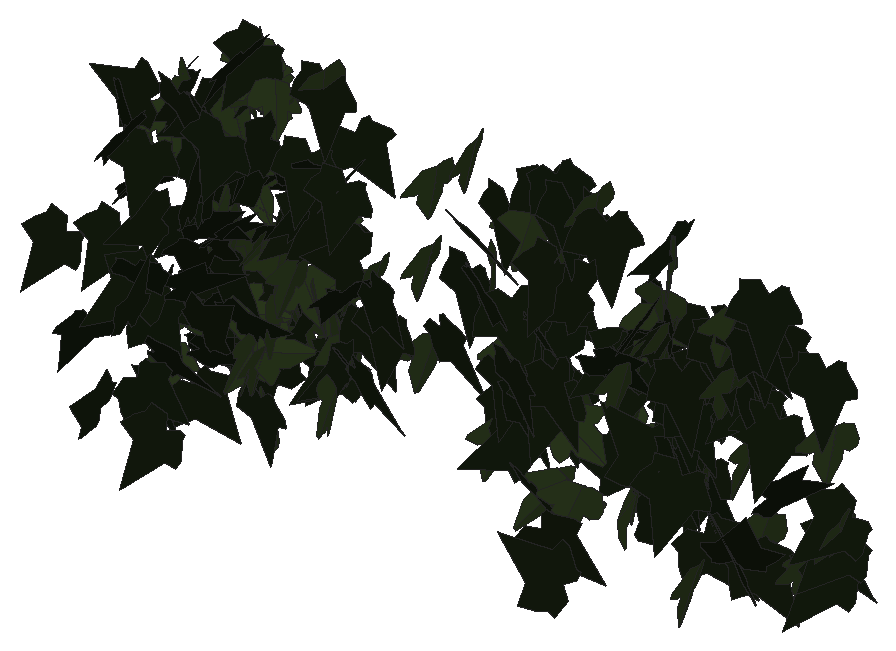
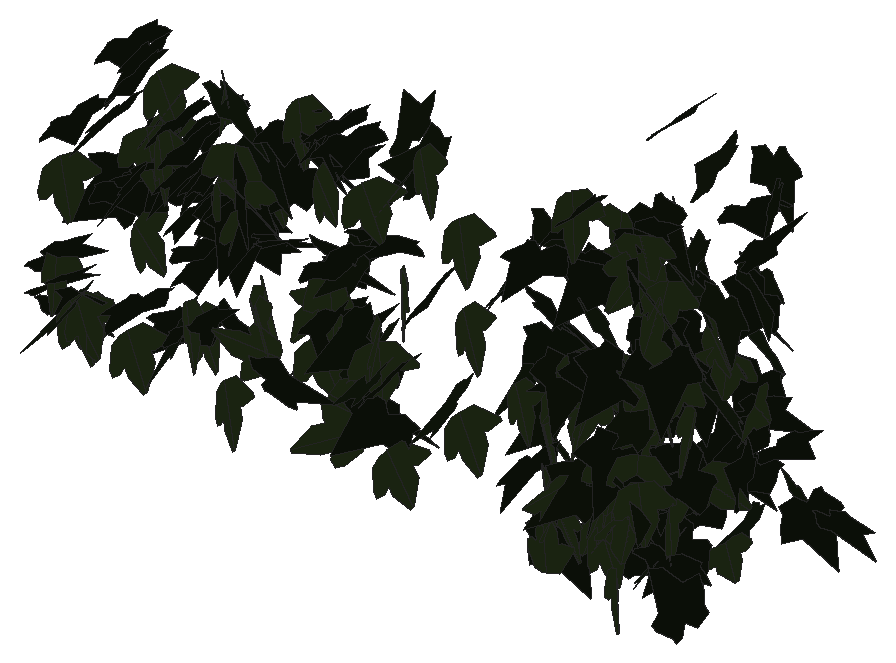
# SketchUp Ruby script. Lengths in inches.
U = 1.inch
M = Sketchup.active_model
def pt(a) = Geom::Point3d.new(a.map { |v| v * U })
def face(e, loops, mat)
  f = e.add_face(loops[0].map { |a| pt(a) })
  loops[1..].each { |l| e.add_face(l.map { |a| pt(a) }).erase! }
  f.material = f.back_material = mat if mat
  f
end
# faces: each face lists its corners as indices into pts; further lists are holes
def faces(e, pts, list, mat = nil) = list.each { |f| face(e, (f[0].is_a?(Array) ? f : [f]).map { |l| l.map { |i| pts[i] } }, mat) }
# xy, xz, yz: faces in a plane at the given z, y or x. An outline is a flat list of corners, or four numbers for a rectangle; further outlines are holes
def ring(l) = l.size == 4 ? [[l[0], l[1]], [l[2], l[1]], [l[2], l[3]], [l[0], l[3]]] : l.each_slice(2).to_a
def flat(e, list, mat, &to3) = list.each { |f| face(e, (f[0].is_a?(Array) ? f : [f]).map { |l| ring(l).map { |u, v| to3.(u, v) } }, mat) }
def xy(e, z, list, mat = nil) = flat(e, list, mat) { |x, y| [x, y, z] }
def xz(e, y, list, mat = nil) = flat(e, list, mat) { |x, z| [x, y, z] }
def yz(e, x, list, mat = nil) = flat(e, list, mat) { |y, z| [x, y, z] }
def lines(e, pts, list) = list.each { |a, b| e.add_line(pt(pts[a]), pt(pts[b])) }
# prism: a flat outline (further loops are holes) pulled along v
def prism(e, loops, v, mat = nil)
  f = face(e, loops, mat); d = Geom::Vector3d.new(v.map { |x| x * U })
  f.pushpull(f.normal.samedirection?(d) ? d.length : -d.length)
end
def box(e, o, s, mat = nil) = prism(e, [[o, [o[0] + s[0], o[1], o[2]], [o[0] + s[0], o[1] + s[1], o[2]], [o[0], o[1] + s[1], o[2]]]], [0, 0, s[2]], mat)
def at(x, y, z, deg = 0) = Geom::Transformation.translation(pt([x, y, z])) * Geom::Transformation.rotation(ORIGIN, Z_AXIS, deg.degrees)
def axes(o, x, y, z) = Geom::Transformation.new([*x, 0, *y, 0, *z, 0, *pt(o).to_a, 1])
def part(name) = M.definitions.add(name)
# library, detail: a bought-in or finely detailed component or shape, given as its bounding box
def library(name, o, s) = part(name).tap { |d| box(d.entities, o, s) }
def detail(e, o, s) = box(e.add_group.entities, o, s)
def put(e, d, t, mat = nil) = e.add_instance(d, t).tap { |i| i.material = mat if mat }
def group(e, t, mat = nil) = e.add_group.tap { |g| g.transformation = t; g.material = mat if mat }.entities
root = M.entities
M.materials.add("efeu1").color = [18, 25, 13]
M.materials.add("efeu2").color = [43, 57, 29]
c1 = part("ivyleaf_9")
p = [[1.54,2.16,1.25],[1.36,2.04,1.19],[-0.21,0.99,0.68],[-0.71,1.11,0.82],[-0.85,0.86,0.67],[-0.8,0.17,0.21],
  [-0.9,-0.01,0.1],[-0.67,-0.16,-0.02],[-0.08,-0.08,-0.05],[-0.03,-0.6,-0.4],[0.65,-0.88,-0.66],[0.83,-0.6,-0.49],
  [1.29,-0.42,-0.43],[1.8125,-0.07,-0.26],[1.21,0.44,0.15]]
faces(c1.entities,p,[[0,1,2,3,4,5,6,7,8,9,10,11,12,13,14]],"efeu1")
c2 = part("ivyleaf_10")
p = [[0,0.5,-0.03],[-0.0625,2.02,-0.43],[-0.19,2.01,-0.46],[-0.54,1.05,-0.29],[-0.52,0.625,-0.18],[-0.83,0.76,-0.28],
  [-1.16,0.64,-0.33],[-1.15,0.33,-0.24],[-0.77,-0.39,0.02],[-0.3,-0.51,0.16],[0.04,-0.48,0.23],[-0.02,2.01,-0.4375],
  [-0.06,2.01,-0.43],[0.04,-0.49,0.23],[0.67,-0.49,0.14],[1.38,0.36,-0.2],[1.375,0.51,-0.24],[0.81,0.65,-0.19],
  [0.62,0.59,-0.15],[0.6,1.09,-0.28],[0.5,1.23,-0.31]]
faces(c2.entities,p,[[0,1,2,3,4,5,6,7,8,9,10],[11,12,0,13,14,15,16,17,18,19,20]],"efeu2")
put(root,c1,axes([2.38,221.57,243.66],[-0.44883,-0.12115,-0.04461],[0.04538,0.00913,-0.45018],[0.13117,-0.41769,0.0031]))
put(root,c2,axes([3.58,222.25,245.79],[-0.02282,0.31345,-0.31292],[-0.01067,-0.3015,-0.32594],[-0.46912,-0.00839,0.02263]))
put(root,c1,axes([3.82,220.47,242.92],[-0.00565,0.32008,-0.30631],[0.01893,-0.29415,-0.33279],[-0.46938,-0.01571,-0.00974]))
put(root,c1,axes([3.92,221.19,244.42],[-0.23643,-0.35754,0.12069],[-0.05224,-0.10638,-0.43577],[0.4026,-0.22377,0.01433]))
put(root,c2,axes([4.58,222.32,246.94],[-0.13824,0.10281,0.41894],[-0.42529,0.10517,-0.15805],[-0.14397,-0.40938,0.06461]))
put(root,c2,axes([4.21,222.22,246.49],[0.43273,0.13992,0.09924],[0.09551,0.03618,-0.44135],[-0.156,0.41029,0.00508]))
put(root,c1,axes([4.64,221.82,247.36],[-0.08663,0.41338,0.1135],[-0.02945,0.10586,-0.43788],[-0.4608,-0.08448,0.00665]))
put(root,c1,axes([4.85,221.9,247.14],[-0.29901,0.33234,0.04787],[-0.02666,0.03934,-0.44981],[-0.36138,-0.27789,-0.00643]))
put(root,c1,axes([4.93,220.75,247.68],[-0.07576,-0.41549,-0.11238],[0.01633,-0.11181,0.43692],[-0.46336,0.06399,0.03377]))
put(root,c1,axes([4.46,223.21,241.59],[-0.00786,-0.11862,0.48566],[0.37542,-0.32217,-0.07261],[0.33015,0.36351,0.09413]))
put(root,c1,axes([5.16,219.1,242.17],[-0.24445,0.31807,0.19958],[-0.11,0.16297,-0.40586],[-0.38582,-0.24798,-0.01074]))
put(root,c2,axes([4.87,221.46,242.12],[0.18139,0.37992,-0.1343],[-0.05106,-0.12028,-0.43197],[-0.43035,0.17441,-0.00535]))
put(root,c1,axes([5.08,220.65,243.03],[-0.00146,-0.05257,0.44908],[0.14124,0.41179,0.05256],[-0.44806,0.12998,0.0151]))
put(root,c2,axes([4.97,222.91,243.27],[0.16507,-0.45863,0.11138],[0.16192,-0.05581,-0.46975],[0.44332,0.19116,0.1301]))
put(root,c1,axes([5.42,221.15,244.96],[-0.17381,0.37113,0.28645],[-0.22198,0.20393,-0.39892],[-0.41293,-0.26585,0.09387]))
put(root,c1,axes([5.3125,220.32,244.26],[-0.39403,-0.23092,0.2035],[-0.18567,-0.08533,-0.45634],[0.24549,-0.43519,-0.01851]))
put(root,c1,axes([4.93,223,242.6],[-0.24815,-0.29365,-0.31968],[0.27813,0.17515,-0.37679],[0.33327,-0.36482,0.07641]))
put(root,c2,axes([5.35,221.4,243.29],[0.1724,0.23306,-0.34403],[-0.33805,-0.15425,-0.27011],[-0.27697,0.33334,0.11554]))
put(root,c2,axes([5.12,222.6875,246.01],[-0.43543,-0.20452,-0.13628],[0.13098,0.04149,-0.48075],[0.20795,-0.45437,0.01745]))
put(root,c1,axes([5.28,222.67,246.39],[0.2811,0.35236,-0.2164],[-0.1876,-0.12452,-0.44643],[-0.3685,0.33218,0.0622]))
put(root,c2,axes([5.31,221.98,244.75],[-0.36612,0.32316,0.10736],[-0.08834,0.06211,-0.4882],[-0.32887,-0.37645,0.01162]))
put(root,c1,axes([5.3125,219.49,248.31],[0.26102,-0.08163,-0.36644],[-0.34839,0.14299,-0.26457],[0.17664,0.40264,0.01967]))
put(root,c1,axes([5.25,220.01,246.49],[0.18079,0.35094,0.20286],[0.09269,0.17517,-0.40437],[-0.4236,0.18811,-0.00191]))
put(root,c1,axes([5.5,219.74,246.71],[-0.09877,0.40443,0.13678],[-0.04326,0.12574,-0.43108],[-0.45726,-0.09925,0.01124]))
put(root,c2,axes([5.41,222.99,246.74],[-0.41969,0.19074,-0.04447],[-0.03985,0.02186,0.4502],[0.20732,0.39034,-0.00348]))
put(root,c1,axes([5.08,220.61,242.03],[0.28274,-0.34,0.07419],[0.04798,-0.05583,-0.44627],[0.37211,0.26554,0.00117]))
put(root,c1,axes([5.7,221.52,247.35],[-0.39604,0.29621,0.07354],[-0.08253,0.01206,-0.49299],[-0.29384,-0.40263,0.03935]))
put(root,c2,axes([5.48,223.19,243.73],[-0.28716,-0.34197,0.04141],[-0.02624,-0.03155,-0.4505],[0.37089,-0.267,0.00019]))
put(root,c1,axes([5.38,219.92,244.75],[0.37325,0.22216,-0.14864],[-0.13716,-0.06663,-0.4271],[-0.25016,0.36801,0.0124]))
put(root,c1,axes([5.28,222.01,242.37],[0.41846,0.19665,0.0215],[0.01597,0.01653,-0.45181],[-0.21295,0.38766,0.00836]))
put(root,c1,axes([5.31,220.42,243.72],[0.11413,-0.39475,-0.28486],[-0.08978,0.2705,-0.41082],[0.47845,0.14492,-0.00913]))
put(root,c1,axes([5.24,221.92,243.76],[0.43877,0.19884,0.13397],[0.12528,0.04809,-0.48166],[-0.20443,0.45624,-0.00762]))
put(root,c1,axes([5.23,222.85,242.47],[0.21399,-0.45177,-0.01042],[0.01905,0.02054,-0.49921],[0.45149,0.21326,0.026]))
put(root,c1,axes([5.68,222.74,243.79],[0.02488,0.42017,0.11464],[0.00053,0.11036,-0.4376],[-0.46914,0.02241,0.00559]))
put(root,c2,axes([5.65,223.05,244.18],[-0.34054,-0.2963,-0.04661],[0.02608,0.03972,-0.44981],[0.32259,-0.316,-0.01283]))
put(root,c2,axes([5.78,223.55,242.04],[-0.32013,0.27253,0.17116],[-0.20236,0.03247,-0.40688],[-0.27799,-0.33748,0.09907]))
put(root,c1,axes([5.95,222.47,247.48],[-0.2793,0.2882,0.20614],[-0.14473,0.14606,-0.4027],[-0.34894,-0.29126,0.00203]))
put(root,c2,axes([5.66,222.22,247.33],[-0.23266,-0.43515,-0.08068],[0.1725,-0.00522,-0.46927],[0.40757,-0.2462,0.15255]))
put(root,c1,axes([6.04,219.6875,246.06],[-0.42437,0.15774,0.10372],[-0.09989,0.0373,-0.44035],[-0.17506,-0.40367,-0.00016]))
put(root,c1,axes([5.98,222.08,243.18],[-0.29202,-0.11745,0.33267],[-0.26024,-0.22283,-0.29692],[0.26021,-0.35465,0.07639]))
put(root,c1,axes([5.7,219.59,242.71],[0.05768,-0.17441,-0.41071],[-0.04482,0.394,-0.18681],[0.46409,0.05973,0.033]))
put(root,c1,axes([6.04,220.82,245.02],[0.18318,0.34092,-0.21872],[-0.1369,-0.17097,-0.39455],[-0.41039,0.20921,0.03399]))
put(root,c1,axes([6.11,218.57,248.33],[-0.12026,0.41668,-0.05882],[0.0159,-0.05461,-0.44856],[-0.45387,-0.11233,-0.00013]))
put(root,c2,axes([6,221.93,245.03],[0.30728,-0.32039,-0.07801],[-0.04546,0.06291,-0.4455],[0.35246,0.28743,0.01055]))
put(root,c2,axes([5.74,222.63,245.54],[0.37507,0.10251,0.2507],[0.25048,0.06573,-0.37658],[-0.1315,0.41761,-0.00226]))
put(root,c1,axes([6.31,221.93,242.65],[-0.37067,0.2467,0.10694],[-0.108,0.03667,-0.43863],[-0.26768,-0.3564,0.02889]))
put(root,c1,axes([6.1,221.75,243.6],[0.19313,0.37256,-0.14126],[-0.08671,-0.1119,-0.42913],[-0.4194,0.1947,0.02367]))
put(root,c1,axes([6.01,223.09,244.4],[0.25845,0.36319,-0.00739],[-0.00273,-0.00685,-0.45234],[-0.39231,0.23931,-0.00173]))
put(root,c2,axes([6.08,221.41,245.81],[0.35729,-0.26353,-0.10571],[-0.08777,0.06111,-0.43987],[0.29215,0.34065,-0.00287]))
put(root,c1,axes([5.77,222.62,245.06],[0.49392,-0.07764,0.0039],[0.02128,0.11091,-0.48708],[0.07476,0.48132,0.11287]))
put(root,c2,axes([6.01,222.41,248.33],[0.4375,0.15631,-0.02734],[-0.02266,-0.01864,-0.45146],[-0.16968,0.40552,-0.01022]))
put(root,c1,axes([6.17,218.6875,244.54],[-0.32584,0.29805,-0.10065],[-0.08951,0.05366,0.44059],[0.32639,0.31227,0.02035]))
put(root,c2,axes([6.02,222.76,243.86],[-0.29111,0.33396,-0.07384],[0.04583,-0.05699,-0.44632],[-0.36588,-0.27285,0.00284]))
put(root,c2,axes([6.01,222.84,242.83],[0.16973,0.4053,0.01674],[0.00762,0.01453,-0.45209],[-0.438,0.15731,-0.00138]))
put(root,c1,axes([5.79,221.28,247.45],[0.26936,-0.3165,0.1704],[0.11017,-0.12822,-0.41908],[0.36881,0.26946,0.00073]))
put(root,c1,axes([6.29,221.76,248.57],[-0.20377,0.39759,-0.2245],[0.04549,-0.22694,-0.4432],[-0.45432,-0.20105,0.05632]))
put(root,c2,axes([6.08,222.44,244.23],[-0.10898,0.03132,-0.43885],[-0.02759,-0.43347,-0.02711],[-0.45615,0.01873,0.10648]))
put(root,c1,axes([6.48,221.93,243.47],[-0.29718,0.04316,0.3475],[-0.35892,0.03607,-0.28948],[-0.05975,-0.43135,0.01056]))
put(root,c1,axes([5.88,223.34,243.11],[0.18161,-0.40114,0.006],[0.00559,-0.00409,-0.45235],[0.43324,0.1682,0.00332]))
put(root,c2,axes([6.03,221.69,245.33],[-0.07319,-0.17005,0.41039],[0.18267,-0.37779,-0.1391],[0.4266,0.1326,0.12998]))
put(root,c1,axes([6.26,221.77,246.08],[-0.06048,0.15389,-0.41912],[0.04269,-0.40284,-0.16569],[-0.46393,-0.05713,0.03939]))
put(root,c1,axes([6.11,219.34,247.69],[-0.23779,-0.37229,-0.04821],[0.02855,0.03822,-0.44981],[0.40417,-0.22173,0.00341]))
put(root,c1,axes([6.27,222.46,247.33],[0.15373,-0.09716,0.41538],[-0.127,0.39538,0.14361],[-0.42538,-0.15316,0.10724]))
put(root,c2,axes([6.2,223.05,244.05],[-0.35389,-0.28311,-0.04292],[0.03555,0.02502,-0.45035],[0.30693,-0.32932,0.00267]))
put(root,c1,axes([5.84,219.93,243.15],[0.39874,-0.10404,0.21337],[0.21232,-0.05873,-0.39891],[0.12899,0.41827,-0.00294]))
put(root,c1,axes([6.27,222.29,248.47],[-0.33067,-0.30723,0.03434],[-0.02376,-0.02469,-0.45109],[0.33287,-0.30696,0.00192]))
put(root,c2,axes([6.15,222.3,247.73],[-0.34812,-0.23113,-0.27458],[0.2434,0.12908,-0.41725],[0.26376,-0.42417,0.02264]))
put(root,c1,axes([6.18,220.75,246.96],[-0.31354,-0.12197,-0.31212],[0.32512,0.04729,-0.32284],[0.12924,-0.41486,0.05496]))
put(root,c1,axes([6.52,222.39,241.75],[0.15282,-0.00661,0.42774],[-0.43864,0.06664,0.14644],[-0.07035,-0.42981,0.01613]))
put(root,c1,axes([6.24,222.3,246.71],[-0.14105,0.07933,-0.42357],[0.3248,-0.27607,-0.15622],[-0.30874,-0.32668,0.02916]))
put(root,c1,axes([6.14,220.63,242.28],[-0.01518,-0.22267,-0.38836],[0.06952,0.36844,-0.231],[0.46438,-0.06244,0.02189]))
put(root,c2,axes([6.21,222.19,248.01],[0.27029,0.32136,0.15882],[0.11244,0.11239,-0.42342],[-0.36744,0.27078,-0.01274]))
put(root,c1,axes([6.25,220.61,245.63],[0.32435,0.28092,0.1475],[0.10275,0.10583,-0.42751],[-0.32396,0.31482,0.01209]))
put(root,c1,axes([6.07,220.92,242.88],[0.38112,0.06429,0.25593],[0.25443,0.07604,-0.372],[-0.10355,0.42345,0.02794]))
put(root,c1,axes([6.28,221.27,244.57],[0.27768,-0.25959,-0.24552],[-0.15187,0.19191,-0.37874],[0.34719,0.29156,0.0307]))
put(root,c2,axes([6.47,222.92,242.41],[-0.06303,-0.48642,0.09706],[0.01069,-0.09915,-0.48995],[0.4959,-0.05969,0.0229]))
put(root,c1,axes([6.57,219.17,242.15],[-0.44393,-0.13934,-0.03035],[0.03094,0.00639,-0.45137],[0.15061,-0.41203,0.00326]))
put(root,c1,axes([6.52,222.86,243.82],[0.21707,-0.04547,-0.39842],[-0.37121,0.17506,-0.20915],[0.18921,0.39562,0.04676]))
put(root,c1,axes([6.35,222.65,245.77],[0.32123,0.30332,0.09732],[0.06492,0.07209,-0.44174],[-0.33661,0.30336,0.00767]))
put(root,c1,axes([6.39,220.98,245.28],[0.24152,0.27566,0.26151],[0.08751,0.25028,-0.36029],[-0.39335,0.22494,0.08042]))
put(root,c1,axes([6.59,219.85,246.31],[0.09615,0.06942,0.4369],[-0.05982,0.42742,-0.06125],[-0.45595,-0.04144,0.10017]))
put(root,c2,axes([6.54,222.48,244.24],[-0.22582,-0.37876,0.04704],[0.01017,-0.05668,-0.44844],[0.41184,-0.20628,0.03686]))
put(root,c1,axes([6.26,219.99,244.62],[0.266,0.10392,0.35689],[0.2955,0.2146,-0.27182],[-0.25027,0.36383,0.05838]))
put(root,c2,axes([6.4,222.92,242.79],[0.00165,0.00839,0.45231],[0.29431,-0.33902,0.00581],[0.36618,0.27244,-0.00671]))
put(root,c2,axes([6.6,222.98,242.92],[-0.43604,0.15085,-0.06117],[0.06291,-0.01213,-0.44815],[-0.16316,-0.40783,-0.0093]))
put(root,c1,axes([6.37,219.89,248.57],[0.17828,-0.41207,0.22003],[0.12183,-0.18634,-0.4477],[0.45097,0.21324,0.03396]))
put(root,c2,axes([6.4,221.55,243.53],[0.04472,-0.12992,-0.4296],[0.4659,0.04843,0.02913],[0.04064,-0.41231,0.13879]))
put(root,c1,axes([6.58,220.3,243.72],[-0.11605,0.00969,0.43826],[0.31469,-0.31254,0.08475],[0.32896,0.3024,0.07354]))
put(root,c2,axes([6.93,221.16,242.87],[0.18226,-0.33228,-0.23333],[-0.0802,0.2133,-0.38664],[0.42551,0.18253,0.02706]))
put(root,c1,axes([6.77,220.08,246.54],[-0.10135,0.26328,0.34665],[0.07605,-0.32699,0.28923],[0.45239,0.11396,0.02904]))
put(root,c1,axes([7.21,222.34,242.95],[-0.32925,0.30802,0.03898],[-0.03653,0.01925,-0.45059],[-0.33312,-0.30656,0.01087]))
put(root,c2,axes([6.98,221.17,243.05],[0.07198,0.26015,-0.35589],[-0.11568,-0.32532,-0.2789],[-0.44961,0.12535,0.01479]))
put(root,c1,axes([6.81,223.11,243.4375],[0.46214,0.0608,0.05116],[0.03965,0.08545,-0.44194],[-0.07459,0.42217,0.08208]))
put(root,c2,axes([7.15,221.52,241.25],[-0.19281,0.39223,-0.06158],[-0.0357,0.04999,0.44809],[0.42692,0.18132,0.00966]))
put(root,c2,axes([7.2,223.25,242.8125],[0.36347,-0.1958,-0.20173],[-0.16716,0.11903,-0.40426],[0.24629,0.36975,0.02332]))
put(root,c2,axes([7.15,221.2,243.03],[0.05432,-0.43206,0.00425],[0.00254,-0.00384,-0.45238],[0.46664,0.05032,0.00197]))
put(root,c1,axes([6.75,221.09,243.6],[0.13887,-0.16067,0.39858],[0.38466,-0.16407,-0.19581],[0.23122,0.36945,0.08638]))
put(root,c2,axes([7.04,221.69,248.11],[0.46397,0.00222,0.07104],[0.07267,0.06223,-0.44224],[-0.0129,0.43052,0.06356]))
put(root,c1,axes([7.41,221.08,247.53],[-0.44852,0.12231,-0.04406],[0.04253,-0.01624,-0.45023],[-0.13317,-0.41714,0.00461]))
put(root,c1,axes([7.43,222.37,245.43],[-0.45645,-0.08004,0.06738],[-0.07078,-0.00202,-0.44723],[0.08579,-0.42757,-0.0105]))
put(root,c2,axes([7.2,223.42,243.3],[0.13325,0.01563,-0.43352],[0.10594,0.42142,0.04663],[0.43787,-0.10671,0.12065]))
put(root,c1,axes([6.97,222.49,245.39],[0.15915,-0.03211,-0.42434],[0.14053,0.41483,0.01492],[0.41909,-0.12691,0.15614]))
put(root,c1,axes([7.05,221.34,242.01],[0.09256,-0.41008,0.12179],[0.05061,-0.10967,-0.43507],[0.4578,0.09504,0.02347]))
put(root,c2,axes([7.3,221.27,243.68],[0.11266,-0.17364,-0.40035],[0.00771,0.39719,-0.18432],[0.45603,0.03619,0.10202]))
put(root,c1,axes([7.51,222.96,242.2],[0.14356,0.2054,-0.37406],[-0.22457,-0.2936,-0.25429],[-0.38687,0.24665,0.0088]))
put(root,c2,axes([7.4375,222.5625,245.42],[-0.15753,-0.38954,0.13241],[-0.00522,-0.13349,-0.43054],[0.44257,-0.14023,0.04205]))
put(root,c1,axes([7.5,222.7,245.32],[0.096,0.41126,0.11481],[-0.00054,0.11288,-0.4369],[-0.45989,0.08572,0.02448]))
put(root,c2,axes([7.36,223.45,241.91],[-0.44783,0.03341,0.13222],[0.13689,-0.00996,0.43265],[0.03766,0.4336,-0.00025]))
put(root,c2,axes([7.24,221.3,243.09],[0.00702,-0.13365,-0.43046],[0.30107,0.31904,-0.10259],[0.36058,-0.26378,0.09404]))
put(root,c1,axes([7.76,222.99,242.28],[-0.43965,-0.11009,0.11098],[-0.10517,-0.04819,-0.43806],[0.1279,-0.41807,0.02127]))
put(root,c1,axes([7.8,221.65,246.05],[-0.34907,0.2911,-0.00456],[0.00359,-0.00286,-0.45238],[-0.3144,-0.32323,-0.00011]))
put(root,c2,axes([7.6,222.94,242.38],[-0.17744,0.3943,0.08553],[-0.02459,0.07959,-0.44413],[-0.43431,-0.1656,-0.0098]))
put(root,c2,axes([7.46,222.66,245.07],[0.25254,0.27149,0.25653],[0.1198,0.22649,-0.36861],[-0.37761,0.25342,0.05462]))
put(root,c2,axes([7.53,221.97,244.3],[0.23183,0.34724,0.15625],[0.03813,0.1536,-0.42166],[-0.40683,0.21227,0.04952]))
put(root,c2,axes([7.67,221.49,244.79],[-0.03288,-0.40682,0.15702],[0.02916,-0.15284,-0.42262],[0.46774,-0.01907,0.03739]))
put(root,c2,axes([7.6,222.82,243.22],[-0.10927,0.42292,-0.01172],[0.0032,-0.01088,-0.45225],[-0.4569,-0.10122,-0.00037]))
put(root,c2,axes([7.74,222.23,248.41],[-0.11326,-0.48158,-0.07247],[0.00618,0.07298,-0.49461],[0.48696,-0.11293,-0.01058]))
put(root,c2,axes([7.73,222.04,244.07],[-0.24509,0.35957,0.09551],[-0.07269,0.06599,-0.44165],[-0.39416,-0.23575,0.02206]))
put(root,c2,axes([7.74,222.2,245.04],[-0.44517,-0.12121,-0.07077],[0.06566,0.03431,-0.44654],[0.13501,-0.41636,-0.01619]))
put(root,c1,axes([7.65,221.55,246.78],[0.39545,0.22792,0.05892],[0.04438,0.04114,-0.44834],[-0.24973,0.36822,0.01362]))
put(root,c1,axes([7.96,221.97,245.72],[-0.45427,0.01655,-0.11408],[0.11496,-0.06084,-0.43406],[-0.03371,-0.43041,0.05697]))
put(root,c1,axes([7.71,222.37,248.24],[0.00576,-0.49847,0.03866],[0.00416,-0.03862,-0.49849],[0.49995,0.00606,0.0037]))
put(root,c1,axes([7.89,221.67,247.11],[-0.32256,-0.28007,-0.15279],[0.13867,0.07729,-0.4247],[0.31215,-0.32374,0.03078]))
put(root,c2,axes([7.94,222.77,244.05],[0.27789,-0.41497,-0.02415],[-0.00533,0.02549,-0.49932],[0.41563,0.27777,0.00975]))
put(root,c2,axes([7.875,222.49,242.91],[0.00413,-0.4268,0.08734],[0.14318,-0.07885,-0.423],[0.44743,0.02917,0.13455]))
put(root,c2,axes([8.08,222.58,242.91],[0.31848,-0.31,-0.08165],[-0.00103,0.10594,-0.43878],[0.34537,0.28618,0.07399]))
put(root,c1,axes([8.01,219.07,248.65],[-0.12399,-0.44497,0.19138],[0.05564,-0.20933,-0.45065],[0.48118,-0.09045,0.10143]))
put(root,c1,axes([8.14,222.93,243.41],[0.12414,-0.42358,-0.23488],[-0.04823,0.23046,-0.44109],[0.48194,0.13217,0.01636]))
put(root,c1,axes([8.67,221.625,243.08],[-0.39706,0.23151,0.0223],[-0.01956,0.01148,-0.45185],[-0.25034,-0.3681,-0.00007]))
put(root,c2,axes([8.49,222.82,244.54],[0.02585,-0.43422,-0.01054],[-0.01565,0.00934,-0.45204],[0.46883,0.02426,-0.01451]))
put(root,c1,axes([8.33,222.45,247.36],[-0.04597,-0.26031,-0.35974],[0.07533,0.33891,-0.27417],[0.46144,-0.08126,0.00892]))
put(root,c1,axes([9.15,221.41,245.56],[-0.33767,0.17792,0.25435],[-0.23557,0.11103,-0.374],[-0.22628,-0.3811,0.00979]))
put(root,c1,axes([8.98,221.25,244.93],[-0.02059,0.40693,-0.15863],[-0.06469,-0.15368,-0.41862],[-0.46487,0.00337,0.06528]))
put(root,c1,axes([9.02,221.22,247.16],[-0.17336,0.40402,0.01578],[-0.02317,0.00779,-0.45178],[-0.43603,-0.16105,0.01773]))
put(root,c1,axes([8.83,221.43,243.43],[0.4371,-0.15922,-0.00881],[-0.00841,0.00335,-0.45231],[0.172,0.4048,0.00028]))
put(root,c1,axes([9,221.28,247.06],[-0.14791,-0.40968,0.05338],[0.02748,-0.06235,-0.44695],[0.44506,-0.1323,0.04534]))
put(root,c2,axes([9.26,220.51,243.2],[0.34912,-0.33136,-0.13535],[-0.07727,0.11483,-0.48046],[0.34949,0.35639,0.02897]))
put(root,c2,axes([9.77,222.79,243.47],[-0.12928,-0.46601,0.12696],[-0.01658,-0.12707,-0.4833],[0.48271,-0.12917,0.0174]))
put(root,c2,axes([9.86,222.57,245.44],[0.04833,-0.49676,0.02984],[0.00137,-0.02985,-0.49911],[0.49766,0.04833,-0.00152]))
put(root,c1,axes([9.79,220.68,243.82],[0.4158,-0.23238,-0.15203],[-0.11449,0.10595,-0.47505],[0.253,0.42985,0.0349]))
put(root,c2,axes([10.07,222.49,247.15],[-0.09101,-0.49159,-0.00778],[-0.00197,0.00827,-0.49993],[0.49164,-0.09096,-0.00344]))
put(root,c1,axes([10.02,222.76,243.85],[0.34419,-0.3522,-0.08656],[-0.02583,0.09523,-0.49017],[0.36176,0.34189,0.04736]))
put(root,c1,axes([10.27,220.5,245.72],[0.33005,-0.3115,-0.20984],[-0.13793,0.1593,-0.45343],[0.34935,0.3572,0.01922]))
put(root,c1,axes([10.49,220.64,245.13],[-0.00698,-0.47016,0.17],[0.04622,-0.1699,-0.46797],[0.49781,0.00919,0.04584]))
put(root,c2,axes([11.08,222.29,248.125],[0.09954,-0.48817,-0.04219],[-0.00688,0.04166,-0.49821],[0.48994,0.09976,0.00158]))
put(root,c1,axes([10.93,222.42,245.5],[0.07453,-0.47612,0.13326],[0.00431,-0.13413,-0.48165],[0.4944,0.07294,-0.01589]))
put(root,c2,axes([11.32,222.88,242.22],[-0.14836,-0.43772,0.19075],[-0.00677,-0.1978,-0.45916],[0.47743,-0.13883,0.05276]))
put(root,c2,axes([11.29,222.6,245.74],[0.29351,-0.38472,-0.12586],[0.0105,0.16265,-0.47269],[0.40465,0.27483,0.10356]))
put(root,c2,axes([11.81,222.67,244.12],[-0.37902,-0.32159,0.05407],[0.03712,-0.12492,-0.48272],[0.32398,-0.36191,0.11857]))
put(root,c1,axes([11.52,222.83,243.08],[-0.04936,-0.16243,-0.4703],[0.25648,0.39667,-0.16392],[0.42636,-0.25743,0.04416]))
put(root,c1,axes([11.67,222.73,243.625],[-0.03848,-0.47102,0.16328],[0.00061,-0.16381,-0.4724],[0.49852,-0.03616,0.01318]))
put(root,c2,axes([11.89,222.65,244.51],[-0.28092,0.41308,-0.02121],[-0.03268,-0.04772,-0.49664],[-0.41233,-0.27765,0.05381]))
put(root,c1,axes([11.83,222.37,247.15],[0.05164,-0.44323,0.22556],[0.03745,-0.22266,-0.44612],[0.49591,0.06297,0.0102]))
put(root,c1,axes([11.75,222.75,243.85],[0.3308,-0.37322,-0.03578],[0.03186,0.07553,-0.49324],[0.37357,0.32404,0.07375]))
put(root,c1,axes([12.4375,222.1,242.75],[-0.46854,0.06518,0.16194],[-0.16183,0.01169,-0.47294],[-0.06544,-0.4956,0.01014]))
put(root,c2,axes([12.3125,222.39,247.07],[-0.24664,-0.40357,0.16216],[0.00298,-0.18799,-0.46331],[0.43492,-0.22757,0.09513]))
put(root,c1,axes([11.89,221.11,247.28],[0.32187,-0.31245,0.22086],[0.20653,-0.10109,-0.44399],[0.3221,0.37704,0.06398]))
put(root,c1,axes([12.4,221.94,243.75],[0.27547,-0.41663,-0.02326],[-0.01368,0.01883,-0.49946],[0.41705,0.2758,-0.00103]))
put(root,c1,axes([12.53,221.59,245.82],[-0.1473,-0.37975,-0.28998],[0.29693,0.16499,-0.3669],[0.37435,-0.28029,0.17691]))
put(root,c1,axes([12.79,222.32,248.06],[-0.05653,-0.46078,-0.1857],[0.02955,0.18345,-0.46419],[0.49591,-0.06346,0.00649]))
put(root,c1,axes([12.63,222.08,243.95],[0.47523,-0.13347,0.07962],[0.07492,-0.0277,-0.49358],[0.13616,0.48106,-0.00633]))
put(root,c1,axes([12.88,221.8,245.41],[0.42994,-0.25436,-0.02131],[-0.0165,0.01396,-0.49953],[0.25472,0.43024,0.00361]))
put(root,c1,axes([13.11,222.49,245.53],[-0.19731,-0.45735,0.04353],[-0.00729,-0.04425,-0.49798],[0.45936,-0.19715,0.0108]))
put(root,c2,axes([12.95,222.15,241.9],[0.15205,0.01343,0.47613],[0.31044,0.37627,-0.10975],[-0.36126,0.329,0.10608]))
put(root,c2,axes([13.37,221.78,242.27],[-0.08228,-0.29293,0.39677],[-0.06696,-0.39189,-0.30321],[0.48862,-0.10303,0.02526]))
put(root,c1,axes([13.68,221.71,245.07],[-0.33638,0.18876,0.31814],[-0.30144,0.10939,-0.38363],[-0.21443,-0.44989,0.0402]))
put(root,c1,axes([13.06,222.23,248.25],[0.11058,-0.44585,-0.19746],[0.03655,0.20948,-0.45253],[0.48625,0.08565,0.07892]))
put(root,c2,axes([13.39,222.3,246.89],[0.12337,-0.44443,0.19304],[0.09363,-0.17358,-0.45946],[0.47541,0.14952,0.0404]))
put(root,c1,axes([13.3125,222.01,244.18],[-0.02789,-0.45416,-0.20727],[0.01251,0.2069,-0.45501],[0.49906,-0.03057,-0.00018]))
put(root,c1,axes([13.19,220,246.92],[0.02189,-0.28497,0.41026],[0.18721,-0.37604,-0.27119],[0.46311,0.16548,0.09024]))
put(root,c2,axes([13.67,221.8,244.43],[-0.46871,0.04881,0.16713],[-0.16981,-0.02215,-0.46976],[-0.03845,-0.49712,0.03734]))
put(root,c1,axes([13.35,222.2,247.88],[0.05518,-0.49475,0.04671],[-0.00654,-0.04771,-0.49768],[0.4969,0.05431,-0.01174]))
put(root,c1,axes([13.56,221.61,246.9],[-0.17431,-0.45171,0.12481],[-0.02106,-0.12548,-0.48354],[0.46816,-0.17382,0.02472]))
put(root,c1,axes([13.78,222.32,247.65],[-0.48414,-0.03926,-0.1186],[0.1182,0.00971,-0.48573],[0.04044,-0.49836,-0.00012]))
put(root,c1,axes([13.45,220.99,242.68],[0.25651,-0.33988,0.26207],[0.20762,-0.16894,-0.42232],[0.37563,0.32548,0.05446]))
put(root,c1,axes([13.55,220.32,245.44],[0.22202,-0.41556,0.16738],[0.06566,-0.15461,-0.47094],[0.44317,0.2311,-0.01408]))
put(root,c1,axes([13.85,221.21,244.71],[-0.22391,-0.447,0.00728],[-0.00307,-0.0066,-0.49995],[0.44705,-0.22393,0.00021]))
put(root,c2,axes([13.9375,222.21,248.11],[-0.04164,-0.49677,-0.03852],[0.00602,0.03815,-0.49851],[0.49823,-0.04198,0.00281]))
put(root,c1,axes([14.33,222.61,242.73],[-0.27937,0.10978,0.39988],[-0.37384,0.14197,-0.30015],[-0.17944,-0.46668,0.00276]))
put(root,c1,axes([13.76,221.23,244.96],[0.1069,-0.4643,-0.15164],[-0.00542,0.15409,-0.47563],[0.48841,0.10334,0.02791]))
put(root,c1,axes([14.43,221.26,246.8],[-0.44497,0.18924,0.12723],[-0.12181,0.03858,-0.4834],[-0.19277,-0.46119,0.01177]))
put(root,c2,axes([14,221.37,243.92],[0.17433,0.34979,0.31186],[0.14367,0.27683,-0.3908],[-0.44606,0.22587,-0.004]))
put(root,c2,axes([14.34,221.2,242.68],[-0.32897,-0.31726,0.2028],[-0.09098,-0.19434,-0.45161],[0.36538,-0.33403,0.07013]))
put(root,c1,axes([14.24,222.13,247.75],[-0.11145,-0.45652,-0.17079],[0.04548,0.1647,-0.4699],[0.48529,-0.12027,0.00482]))
put(root,c1,axes([14.73,222.32,245.2],[-0.41435,-0.21616,0.17773],[-0.06105,-0.24007,-0.43433],[0.27311,-0.38163,0.17255]))
put(root,c2,axes([14.58,222.54,243.87],[0.26362,-0.42102,0.05694],[0.04668,-0.0379,-0.49637],[0.42228,0.26702,0.01933]))
put(root,c1,axes([14.36,220.22,242.41],[-0.02854,-0.04897,-0.49678],[0.31628,0.3832,-0.05594],[0.3862,-0.31743,0.0091]))
put(root,c2,axes([14.4375,222.6,243.23],[0.14515,0.01454,-0.47825],[0.47219,0.07635,0.14564],[0.07727,-0.49392,0.00844]))
put(root,c1,axes([15.12,219.71,241.85],[-0.20073,-0.45215,-0.0726],[-0.02887,-0.06662,0.4947],[-0.45703,0.2028,0.00064]))
put(root,c1,axes([14.97,222.35,245.23],[-0.37071,-0.3189,-0.1043],[0.11864,0.0208,-0.48527],[0.31385,-0.38454,0.06025]))
put(root,c2,axes([15.08,222.36,245.53],[-0.14485,-0.44279,-0.18153],[0.05317,0.1736,-0.46587],[0.4756,-0.15427,-0.0032]))
put(root,c1,axes([15.16,222.35,245.7],[0.21012,0.42398,-0.16153],[-0.0553,-0.15275,-0.47287],[-0.45032,0.21659,-0.0173]))
put(root,c1,axes([15.4,222.27,246.05],[-0.46804,0.17242,0.0348],[-0.03828,-0.0033,-0.49852],[-0.17168,-0.46932,0.01629]))
put(root,c2,axes([15.18,222.73,242.17],[0.05591,-0.49496,-0.04347],[-0.00046,0.04369,-0.49809],[0.49686,0.05574,0.00443]))
put(root,c1,axes([15.15,222.3,245.82],[0.29215,0.40033,-0.0662],[-0.04674,-0.04783,-0.49551],[-0.40306,0.29572,0.00947]))
put(root,c1,axes([15.41,222.28,246.44],[0.12476,0.00436,-0.48417],[-0.48415,0.0068,-0.1247],[0.0055,0.49993,0.00592]))
put(root,c2,axes([15.26,222.31,246.11],[0.42755,0.21146,-0.14996],[-0.18059,0.03545,-0.4649],[-0.18598,0.45169,0.10669]))
put(root,c1,axes([15.16,220.79,245.9375],[0.45787,0.19324,0.05487],[0.05308,0.01535,-0.49694],[-0.19375,0.46089,-0.00646]))
put(root,c2,axes([15.49,222.24,246.65],[-0.49426,-0.0266,0.07068],[-0.0706,-0.00344,-0.49498],[0.02682,-0.49928,-0.00035]))
put(root,c1,axes([15.57,221.44,246.53],[-0.27861,0.37248,-0.1834],[0.10446,-0.15087,-0.46511],[-0.40182,-0.29749,0.00625]))
put(root,c2,axes([15.36,221.71,243.4],[0.25973,-0.37855,0.19809],[0.14552,-0.13958,-0.45754],[0.4017,0.29533,0.03767]))
put(root,c1,axes([15.78,222.11,247.82],[-0.33516,0.37075,0.01444],[-0.06003,-0.03498,-0.49515],[-0.36614,-0.33365,0.06797]))
put(root,c2,axes([15.56,222.29,246.02],[0.02485,-0.49938,0.00182],[-0.00777,-0.00221,-0.49993],[0.49932,0.02482,-0.00787]))
put(root,c2,axes([15.59,220.97,245.74],[0.00046,-0.49512,0.06968],[0.00145,-0.06967,-0.49512],[0.5,0.00066,0.00137]))
put(root,c2,axes([15.42,221.16,242.68],[0.18538,-0.31859,-0.33784],[0.20106,-0.27283,0.36761],[-0.41858,-0.27215,0.02695]))
put(root,c1,axes([16,221.5,242.57],[-0.05469,0.13008,0.47968],[-0.32707,0.35392,-0.13327],[-0.37421,-0.32836,0.04638]))
put(root,c2,axes([15.79,222.09,247.79],[-0.24503,0.35027,-0.25937],[0.01335,-0.29137,-0.40611],[-0.43564,-0.20594,0.13343]))
put(root,c1,axes([15.92,222.47,244.55],[0.00001,-0.49343,-0.08079],[-0.00367,0.08079,-0.49342],[0.49999,0.0006,-0.00362]))
put(root,c1,axes([16.07,222.64,243.25],[-0.15576,-0.47378,0.03565],[0.00669,-0.0397,-0.49838],[0.47507,-0.15477,0.01871]))
put(root,c2,axes([16.23,222.5,243.31],[0.13963,-0.45917,-0.14025],[-0.03653,0.13547,-0.47991],[0.47872,0.14427,0.00429]))
put(root,c1,axes([16.18,222.35,244.66],[-0.30018,-0.39949,0.01733],[0.02155,-0.0378,-0.4981],[0.39928,-0.2983,0.03991]))
put(root,c1,axes([16.55,220.5625,244.43],[-0.42534,-0.19916,-0.17154],[-0.15583,-0.07172,0.46965],[-0.21168,0.45298,-0.00106]))
put(root,c1,axes([16.17,222.38,245.5],[0.11666,-0.47568,-0.10057],[-0.0001,0.10341,-0.48919],[0.4862,0.11415,0.02404]))
put(root,c1,axes([16.47,222.33,242.99],[0.36221,-0.263,-0.22278],[-0.17386,0.13964,-0.44752],[0.29762,0.40166,0.00971]))
put(root,c1,axes([16.6,222.16,246.52],[-0.01601,-0.49839,0.03673],[-0.00038,-0.03673,-0.49865],[0.49974,-0.01599,0.0008]))
put(root,c1,axes([16.8,221.12,245.52],[0.09602,-0.49064,-0.00726],[-0.00693,0.00605,-0.49992],[0.49064,0.09611,-0.00563]))
put(root,c1,axes([16.79,221.93,245.85],[0.18563,-0.40252,-0.23135],[-0.04411,0.23273,-0.44033],[0.46216,0.18389,0.05089]))
put(root,c1,axes([16.86,221.14,245.53],[0.16894,-0.43289,-0.18456],[-0.05668,0.17595,-0.46457],[0.46717,0.17789,0.01038]))
put(root,c2,axes([17.09,222.21,246.26],[0.13841,-0.47832,-0.04535],[0.03259,0.05643,-0.49574],[0.47936,0.13427,0.0468]))
put(root,c1,axes([16.83,220.88,244.5625],[0.22281,-0.44604,0.0375],[0.01037,-0.03673,-0.49854],[0.44749,0.22294,-0.00712]))
put(root,c2,axes([17.15,220.98,242.15],[0.11336,-0.47801,0.09305],[0.02651,-0.08934,-0.49124],[0.48626,0.11631,0.00509]))
put(root,c1,axes([16.9375,221.61,242.6],[0.03243,-0.3019,-0.39724],[0.17303,0.38018,-0.27481],[0.46798,-0.11965,0.12913]))
put(root,c1,axes([17.07,220.75,246.31],[0.01973,-0.48957,-0.09966],[-0.00948,0.09936,-0.48994],[0.49952,0.02123,-0.00536]))
put(root,c1,axes([17.1,221.77,246.68],[0.06402,-0.49301,-0.0533],[0.00114,0.05389,-0.49709],[0.49588,0.06352,0.00802]))
put(root,c2,axes([17.35,222.75,242.46],[-0.15882,-0.45746,0.12454],[-0.00104,-0.13101,-0.48253],[0.47411,-0.15353,0.04066]))
put(root,c1,axes([17.18,222.09,246.85],[0.2202,-0.4489,-0.00154],[0.00134,0.00237,-0.49999],[0.4489,0.2202,0.00225]))
put(root,c2,axes([17.51,221.67,247.1875],[-0.12602,-0.45875,0.15385],[0.01408,-0.16239,-0.47269],[0.48365,-0.11481,0.05385]))
put(root,c2,axes([17.52,222.09,246.23],[-0.35848,-0.33775,0.08611],[0.00874,-0.1322,-0.48213],[0.34845,-0.34416,0.10069]))
put(root,c1,axes([17.44,220.24,244.55],[-0.29285,-0.40107,-0.05815],[0.03431,0.04695,-0.49661],[0.40381,-0.29486,0.00003]))
put(root,c2,axes([17.54,222.2,244.37],[0.08607,-0.44421,0.21276],[0.02845,-0.21114,-0.45234],[0.49171,0.08997,-0.01107]))
put(root,c2,axes([17.65,221.43,246.17],[-0.041,-0.49686,0.03801],[-0.00405,-0.03781,-0.49855],[0.4983,-0.04119,-0.00092]))
put(root,c1,axes([17.71,222.22,245.57],[-0.34026,-0.31645,0.18462],[-0.06084,-0.19966,-0.45435],[0.36128,-0.33166,0.09737]))
put(root,c1,axes([17.54,222.14,245.6875],[0.2795,-0.31053,-0.27468],[-0.10862,0.26485,-0.40995],[0.4001,0.28883,0.08059]))
put(root,c1,axes([18.18,222.05,245.14],[-0.23441,-0.43956,-0.04293],[0.00647,0.04519,-0.49791],[0.4416,-0.23398,-0.0155]))
put(root,c1,axes([18.14,221.7,247.21],[0.0448,-0.49633,0.04059],[-0.0005,-0.0408,-0.49833],[0.49799,0.04461,-0.00415]))
put(root,c1,axes([18.08,221.5625,242.6],[0.11948,-0.40104,-0.27367],[0.06166,0.29208,-0.40111],[0.48158,0.0621,0.11925]))
put(root,c1,axes([18.11,222.1875,246.74],[0.24971,-0.36025,-0.24055],[-0.03402,0.26049,-0.42543],[0.43184,0.22883,0.10558]))
put(root,c1,axes([18.26,221.7,247.87],[-0.09189,-0.48603,-0.07302],[0.00744,0.0729,-0.4946],[0.49143,-0.09198,-0.00616]))
put(root,c1,axes([18.31,221.1,247.4],[0.22255,-0.32834,-0.30441],[-0.11398,0.2872,-0.3931],[0.43299,0.24436,0.05299]))
put(root,c2,axes([18.77,222.27,242.42],[-0.10734,-0.48819,0.01201],[-0.00229,-0.01179,-0.49986],[0.48834,-0.10736,0.00029]))
put(root,c2,axes([18.82,222.47,242.45],[-0.13075,-0.4458,0.18485],[-0.04263,-0.1801,-0.46449],[0.48072,-0.13722,0.00909]))
put(root,c1,axes([18.79,222.62,242.7],[0.3488,-0.30901,-0.18125],[-0.04959,0.20889,-0.45156],[0.35479,0.33299,0.11507]))
put(root,c1,axes([18.91,220.96,244.36],[0.23021,0.28083,0.34371],[0.19998,0.28003,-0.36275],[-0.39624,0.30449,0.01661]))
put(root,c1,axes([19.1875,219.85,243.3],[0.20064,-0.3871,0.24474],[-0.09839,0.22453,0.43578],[-0.44729,-0.22303,0.01393]))
put(root,c1,axes([19.03,222.37,246.34],[-0.05286,-0.49671,-0.02213],[0.00121,0.02213,-0.49951],[0.4972,-0.05286,-0.00114]))
put(root,c1,axes([19.01,219.84,243.65],[0.46347,0.13058,0.13469],[-0.12977,-0.03608,0.48152],[0.13547,-0.4813,0.00045]))
put(root,c1,axes([19.36,222.29,242.47],[-0.45015,-0.21388,0.04028],[-0.0347,-0.02083,-0.49836],[0.21486,-0.45146,0.00391]))
put(root,c2,axes([19.25,222.32,245.14],[-0.20549,-0.45145,0.06298],[0.02329,-0.07939,-0.49311],[0.45522,-0.19973,0.05366]))
put(root,c1,axes([19.37,222.57,242.9],[-0.30435,-0.33291,0.21575],[-0.02284,-0.25677,-0.42843],[0.39605,-0.27064,0.14108]))
put(root,c1,axes([19.4375,222.53,243.44],[-0.31071,-0.29933,0.25272],[-0.11653,-0.23733,-0.42437],[0.37401,-0.32261,0.07772]))
put(root,c2,axes([19.39,222.29,243.29],[0.00813,-0.47422,-0.15828],[0.03064,0.15848,-0.47323],[0.49899,-0.00201,0.03163]))
